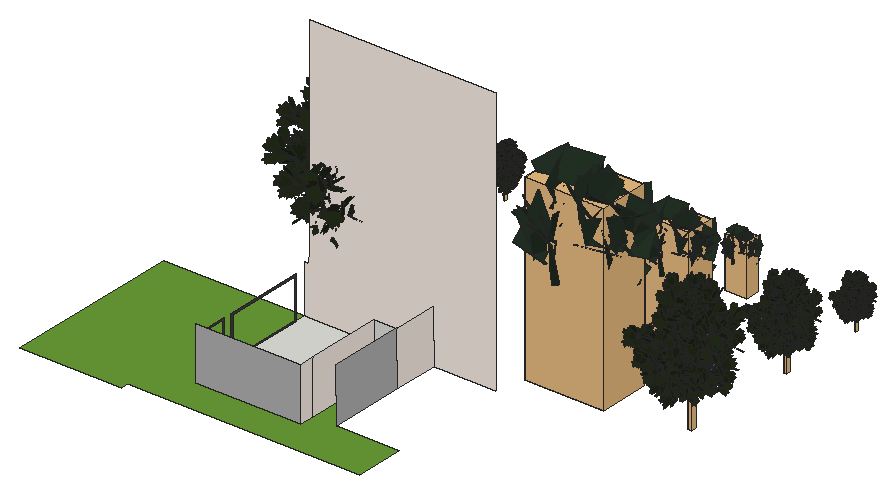
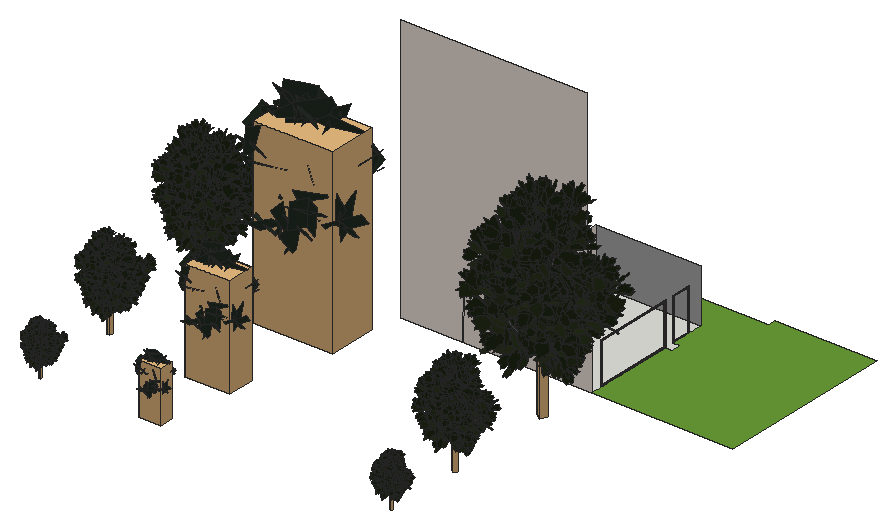
# SketchUp Ruby script. Lengths in inches.
U = 1.inch
M = Sketchup.active_model
def pt(a) = Geom::Point3d.new(a.map { |v| v * U })
def face(e, loops, mat)
  f = e.add_face(loops[0].map { |a| pt(a) })
  loops[1..].each { |l| e.add_face(l.map { |a| pt(a) }).erase! }
  f.material = f.back_material = mat if mat
  f
end
# faces: each face lists its corners as indices into pts; further lists are holes
def faces(e, pts, list, mat = nil) = list.each { |f| face(e, (f[0].is_a?(Array) ? f : [f]).map { |l| l.map { |i| pts[i] } }, mat) }
# xy, xz, yz: faces in a plane at the given z, y or x. An outline is a flat list of corners, or four numbers for a rectangle; further outlines are holes
def ring(l) = l.size == 4 ? [[l[0], l[1]], [l[2], l[1]], [l[2], l[3]], [l[0], l[3]]] : l.each_slice(2).to_a
def flat(e, list, mat, &to3) = list.each { |f| face(e, (f[0].is_a?(Array) ? f : [f]).map { |l| ring(l).map { |u, v| to3.(u, v) } }, mat) }
def xy(e, z, list, mat = nil) = flat(e, list, mat) { |x, y| [x, y, z] }
def xz(e, y, list, mat = nil) = flat(e, list, mat) { |x, z| [x, y, z] }
def yz(e, x, list, mat = nil) = flat(e, list, mat) { |y, z| [x, y, z] }
def lines(e, pts, list) = list.each { |a, b| e.add_line(pt(pts[a]), pt(pts[b])) }
# prism: a flat outline (further loops are holes) pulled along v
def prism(e, loops, v, mat = nil)
  f = face(e, loops, mat); d = Geom::Vector3d.new(v.map { |x| x * U })
  f.pushpull(f.normal.samedirection?(d) ? d.length : -d.length)
end
def box(e, o, s, mat = nil) = prism(e, [[o, [o[0] + s[0], o[1], o[2]], [o[0] + s[0], o[1] + s[1], o[2]], [o[0], o[1] + s[1], o[2]]]], [0, 0, s[2]], mat)
def at(x, y, z, deg = 0) = Geom::Transformation.translation(pt([x, y, z])) * Geom::Transformation.rotation(ORIGIN, Z_AXIS, deg.degrees)
def axes(o, x, y, z) = Geom::Transformation.new([*x, 0, *y, 0, *z, 0, *pt(o).to_a, 1])
def part(name) = M.definitions.add(name)
# library, detail: a bought-in or finely detailed component or shape, given as its bounding box
def library(name, o, s) = part(name).tap { |d| box(d.entities, o, s) }
def detail(e, o, s) = box(e.add_group.entities, o, s)
def put(e, d, t, mat = nil) = e.add_instance(d, t).tap { |i| i.material = mat if mat }
def group(e, t, mat = nil) = e.add_group.tap { |g| g.transformation = t; g.material = mat if mat }.entities
root = M.entities
M.materials.add("Color_D09").color = [86, 59, 49]
M.materials.add("Green ash – green texture").color = [33, 41, 22]
M.materials.add("Niraj_Hair_Gray").color = [178, 178, 178]
M.materials.add("[0009_Linen]").color = [250, 240, 230]
M.materials.add("[Asphalt New]").color = [67, 60, 62]
M.materials.add("[Color_005]1").color = [114, 114, 114]
M.materials.add("[Grass Dark Green]").color = [106, 157, 55]
M.materials.add("euc leaf02").color = [35, 48, 36]
c1 = part("Component\#32")
xz(c1.entities,0,[[2.54,0,9.87,0.64,10.99,2.07,11.4,3.42,15.13,2.28,14.48,4.31,16.14,5.21,16.14,6.08,19.81,7.28,19.6,9.67,17.45,11.49,17.45,12.16,18.82,14.37,17.48,14.37,14.41,13.66,14.41,15.23,12.5625,17.49,9.84,15.21,8.9,13.85,7.74,13.625,7.35,12.68,6.87,13.02,6.35,12.27,5.92,10.47,4.2,7.42,2.84,6.89,0,2.38,0.07,1.59,2.8125,4.94,3.37,3.59,2.54,3.37,2.12,2.22]],"Green ash – green texture")
c2 = part("Component\#31")
xz(c2.entities,0,[[1.1,0,1.61,0,2.73,1.11,4.34,2.72,5.21,6.36,5.85,7.16,6.35,6.9375,6.85,8.05,8.03,8.05,8.625,9.25,10.11,11.7,9.56,13.83,9.56,15.84,7.83,15.84,6.03,14.37,5.31,16.54,4.4375,17.39,1.45,14.31,0,9.15,1.4,5.18,3.01,6.08,1.98,1.39]],"Green ash – green texture")
c3 = part("Component\#30")
put(c3.entities,c1,axes([0,7.77,0],[1,0,0],[0,0.89571,0.44464],[0,-0.44464,0.89571]))
put(c3.entities,c2,axes([2.15,6.37,5.26],[0.57629,-0.80824,0.12095],[0.79263,0.51673,-0.3236],[0.19905,0.28236,0.93843]))
c4 = part("Component\#33")
put(c4.entities,c3,axes([-4.97,-3.22,4.05],[0.69883,-0.69034,0.18725],[0.53248,0.3273,-0.7806],[0.47759,0.64522,0.59632]))
c5 = part("Component\#35")
put(c5.entities,c4,axes([0,5.2,2.2],[1,0,0],[0,0.90259,0.43051],[0,-0.43051,0.90259]))
c6 = part("leaf group 2")
put(c6.entities,c5,axes([-11.99,4.41,-4.35],[2.22014,-0.82385,1.14017],[1.36501,1.77637,-1.37441],[-0.33979,1.75315,1.92841]))
c7 = part("Component\#37")
put(c7.entities,c6,axes([-5.27,11.65,1.68],[-0.48323,0.10636,-0.43072],[-0.11515,-0.64511,-0.03012],[-0.42845,0.05342,0.49388]))
c8 = part("Component\#36")
xz(c8.entities,0,[[0.64,0,0,0.1875,4.21,2.81,8.59,4.11,12.8,4.11,19.57,2.81,12.8,3.73,8.59,3.73,4.21,2.3125]],"Color_D09")
c9 = part("Leaf cluster")
put(c9.entities,c7,axes([23.53,12.57,24.85],[0.06536,-0.90475,-0.42089],[0.61791,-0.2945,0.72901],[-0.78353,-0.30772,0.53981]))
put(c9.entities,c7,axes([22.7,12.25,24.83],[-0.47146,-0.89493,0.11311],[0.80135,-0.48549,-0.35888],[0.36776,-0.0521,0.90651]))
put(c9.entities,c7,axes([24.25,0.65,20.83],[0.8253,-0.50372,0.24924],[0.23848,0.71461,0.65749],[-0.51157,-0.48438,0.71194]))
put(c9.entities,c7,axes([23.54,-2.45,18.63],[0.04689,-0.92492,0.3511],[0.72122,-0.28285,-0.64421],[0.71641,0.2674,0.65188]))
put(c9.entities,c7,axes([22.39,16.15,27.04],[-0.5311,-0.82173,0.2419],[0.41574,0.01583,0.89559],[-0.77461,0.50499,0.40813]))
put(c9.entities,c8,axes([22.76,-5.09,13.48],[0,1.66539,0.44624],[-1.72414,0,0],[0,-0.44624,1.66539]))
c10 = part("Bare twig")
p = [[0,0,0.13],[0.41,0.77,0],[4.07,2.79,10.125],[3.73,2.15,10.23],[7.66,4.77,23.875],[7.4,4.27,23.96],
  [8.6875,5.26,35.99],[8.5,4.91,36.05],[8.32,4.9375,46.95],[8.21,4.74,46.98]]
faces(c10.entities,p,[[0,1,2,3],[3,2,4,5],[4,6,7,5],[6,8,9,7]],"[Color_005]1")
c11 = part("Leafy twig")
put(c11.entities,c10,axes([3.13,0.17,-0.45],[3.38032,6.88592,0.52481],[-5.85488,3.97559,0.303],[0,-1.35912,3.54524]))
put(c11.entities,c7,axes([0.37,31.375,148.94],[0.47772,0.64064,-1.51139],[2.85768,-0.62659,0.20284],[-0.43926,-3.3797,-0.3241]))
c12 = part("Leafy branch")
put(c12.entities,c9,axes([28.11,72.66,46.26],[0.77413,-0.41274,-0.47998],[0.6311,0.56229,0.53435],[0.04934,-0.71657,0.69577]))
put(c12.entities,c9,axes([31.25,3.94,9.17],[0.73236,0.67893,0.05208],[-0.46223,0.55185,-0.69413],[-0.5,0.48428,0.71797]))
put(c12.entities,c9,axes([20.16,84.84,57.95],[0.96628,0.19619,0.16678],[-0.2575,0.73909,0.62245],[-0.00115,-0.6444,0.76469]))
put(c12.entities,c9,axes([30.13,29.18,11.93],[0.86603,0.2796,0.41452],[0,0.82904,-0.55919],[-0.5,0.48428,0.71797]))
put(c12.entities,c9,axes([47.67,28.63,-3.7],[0.1205,-0.71255,0.69119],[0.96646,0.24327,0.08231],[-0.2268,0.65809,0.71797]))
put(c12.entities,c9,axes([48.76,50.64,76.31],[-0.6716,0.46861,-0.57389],[0.01402,0.78248,0.62252],[0.74078,0.41004,-0.53209]))
put(c12.entities,c11,axes([42.34,0,10.34],[0.39368,0,0],[0,0.22544,-0.24092],[0,0.54032,0.50562]))
put(c12.entities,c9,axes([64.51,80.82,101.08],[-0.99604,0.06562,-0.06004],[-0.0106,0.58266,0.81265],[0.08831,0.81006,-0.57966]))
c13 = part("Leafy branch \#2")
put(c13.entities,c9,axes([-3.64,36.17,23.18],[0.95801,0.10249,0.26779],[-0.28581,0.41631,0.86313],[-0.02302,-0.90343,0.42812]))
put(c13.entities,c9,axes([13.16,55.79,39.92],[0.70711,-0.61725,0.34497],[0,0.48786,0.87292],[-0.70711,-0.61725,0.34497]))
put(c13.entities,c11,axes([18.8125,5.17,0.46],[0.25503,0,0],[0,0.20007,-0.0752],[0,0.16866,0.44872]))
put(c13.entities,c9,axes([23.62,-10.17,21.5],[-0.56253,0.81775,0.12181],[0.38738,0.13053,0.91263],[0.73041,0.56057,-0.39021]))
put(c13.entities,c9,axes([45.18,27.18,68.96],[-0.96593,-0.22593,0.12627],[0.12295,0.02876,0.992],[-0.22775,0.97372,0]))
c14 = library("Tree trunk",[-6.35,9.4375,-76.57],[12.56,13.68,315.77])
c15 = part("Leafy branch \#3")
put(c15.entities,c11,axes([21.47,3.93,0.22],[0.25503,0,0],[0,0.21068,-0.03601],[0,0.08077,0.47252]))
put(c15.entities,c9,axes([-4.05,13.6875,55.34],[0.70711,0.70373,-0.069],[0,0.09758,0.99523],[0.70711,-0.70373,0.069]))
put(c15.entities,c9,axes([6.52,33.54,18.07],[0.92587,-0.37604,0.03687],[0,0.09758,0.99523],[-0.37784,-0.92145,0.09035]))
c16 = part("Leafy branch \#1")
put(c16.entities,c9,axes([26.17,74.02,40.56],[0.25882,-0.64004,0.72344],[0,0.74896,0.66262],[-0.96593,-0.1715,0.19384]))
put(c16.entities,c9,axes([6.38,24.03,55.81],[-0.04786,0.8645,-0.50035],[0.15558,0.50126,0.85119],[0.98666,-0.03711,-0.15849]))
put(c16.entities,c11,axes([17.68,0,1.01],[0.32282,0,0],[0,0.21407,-0.16545],[0,0.37107,0.48011]))
put(c16.entities,c9,axes([-9.1875,31.15,28.07],[0.82314,0.37626,-0.42529],[0,0.74896,0.66262],[0.56784,-0.54543,0.61649]))
put(c16.entities,c9,axes([0.54,-12.07,9.94],[0.19622,0.90478,-0.37799],[-0.67396,0.40444,0.61823],[0.71224,0.13344,0.68914]))
put(c16.entities,c9,axes([7.34,9.15,39.57],[0.05153,0.73872,-0.67204],[0.38679,0.60565,0.6954],[0.92072,-0.29578,-0.25452]))
put(c16.entities,c9,axes([36.2,51.23,15.73],[-0.18626,-0.35374,0.91661],[-0.31641,0.90483,0.2849],[-0.93016,-0.23696,-0.28046]))
c17 = part("Tree")
put(c17.entities,c12,axes([209.16,146.26,190.79],[-0.28773,1.46382,-0.87256],[-1.6259,0,0.48096],[0.49836,0.84514,1.51132]))
put(c17.entities,c12,axes([134.38,215.25,141.01],[1.59145,0,0],[0,1.58386,0.23671],[0,-0.32836,1.69393]))
put(c17.entities,c13,axes([178.04,237.71,388.46],[0,-1.63474,0],[1.63474,0,0],[0,0,1.78187]))
put(c17.entities,c12,axes([256.65,171.18,211.31],[-1.36815,1.04036,0],[-1.04036,-1.36815,0],[0,0,1.87346]))
put(c17.entities,c12,axes([167.11,160.33,284.63],[0.63716,1.20925,-0.47341],[-1.25908,0.71729,0.13762],[0.43501,0.34501,1.46674]))
put(c17.entities,c14,axes([199.97,188.06,127.43],[1.59145,0,0],[0,1.59145,0],[0,0,1.66425]))
put(c17.entities,c12,axes([275.77,218.4,281.93],[-1.57517,-0.28132,-0.44593],[0.06295,-1.50318,0.62621],[-0.42383,0.67416,1.53786]))
put(c17.entities,c12,axes([190.14,288,146.64],[0.35111,-1.78964,0],[1.72866,0.33915,0.47202],[-0.50488,-0.09905,1.92016]))
put(c17.entities,c12,axes([257.54,236.65,165.53],[-1.29152,-0.54158,0],[0.54158,-1.29152,0],[0,0,1.52652]))
put(c17.entities,c12,axes([175.36,274.13,265.04],[0.47642,-1.31213,-0.12271],[1.30597,0.45529,0.24003],[-0.16973,-0.17989,1.50253]))
put(c17.entities,c13,axes([228.65,212.14,385.35],[-1.53723,0.39369,-0.12111],[-0.39786,-1.55122,0.00748],[-0.10661,0.11241,1.71849]))
put(c17.entities,c15,axes([179.375,247.82,455.73],[0.79573,-1.37824,0],[1.37824,0.79573,0],[0,0,1.73468]))
put(c17.entities,c15,axes([220.2,190.4,436.52],[-0.90108,1.29724,0.19482],[-1.26794,-0.9219,0.27414],[0.36658,0,1.69551]))
put(c17.entities,c16,axes([195.4,185.625,330.61],[0,1.80471,0],[-1.731,0,0.5105],[0.55644,0,1.88679]))
put(c17.entities,c16,axes([180.07,237.23,322.66],[1.03006,-1.73903,-0.39964],[1.71651,0.8636,0.79163],[-0.4607,-0.67055,2.05597]))
put(c17.entities,c12,axes([252.86,167.09,121.2],[-1.29065,1.04142,0.30989],[-1.03312,-1.28343,0.15838],[0.47872,-0.11505,1.68865]))
put(c17.entities,c12,axes([145.45,238.15,252.03],[1.32497,-0.45364,0],[0.45364,1.32497,0],[0,0,1.52652]))
put(c17.entities,c16,axes([222.54,228.83,294],[-1.20488,-1.04179,0.83261],[1.23186,-1.24114,0.27288],[0.38905,0.70343,1.7146]))
put(c17.entities,c16,axes([223.77,224.36,314.875],[-1.40575,-0.68986,-0.30962],[0.56266,-1.37824,0.6133],[-0.4899,0.39658,1.59284]))
put(c17.entities,c16,axes([166.75,216.1,346.53],[1.65511,0,0],[0,1.6365,0.2475],[0,-0.26977,1.78379]))
put(c17.entities,c13,axes([162.33,209.39,372.71],[1.56679,-0.27909,0],[0.27909,1.56679,0],[0,0,1.73468]))
put(c17.entities,c13,axes([203.35,171.86,386.35],[0.15996,1.63137,0],[-1.63137,0.15996,0],[0,0,1.78672]))
c18 = part("Green Ash")
put(c18.entities,c14,axes([99.99,94.03,63.71],[0.79573,0,0],[0,0.79573,0],[0,0,0.83213]))
put(c18.entities,c13,axes([101.67,85.93,193.17],[0.07998,0.81569,0],[-0.81569,0.07998,0],[0,0,0.89336]))
put(c18.entities,c13,axes([89.02,118.86,194.23],[0,-0.81737,0],[0.81737,0,0],[0,0,0.89093]))
put(c18.entities,c12,axes([137.88,109.2,140.96],[-0.78759,-0.14066,-0.22296],[0.03147,-0.75159,0.31311],[-0.21191,0.33708,0.76893]))
put(c18.entities,c12,axes([67.1875,107.625,70.5],[0.79573,0,0],[0,0.79193,0.11835],[0,-0.16418,0.84696]))
put(c18.entities,c12,axes([104.58,73.13,95.39],[-0.14386,0.73191,-0.43628],[-0.81295,0,0.24048],[0.24918,0.42257,0.75566]))
put(c18.entities,c12,axes([128.33,85.59,105.66],[-0.68407,0.52018,0],[-0.52018,-0.68407,0],[0,0,0.93673]))
put(c18.entities,c12,axes([128.77,118.32,82.77],[-0.64576,-0.27079,0],[0.27079,-0.64576,0],[0,0,0.76326]))
put(c18.entities,c13,axes([114.32,106.07,192.67],[-0.76861,0.19684,-0.06056],[-0.19893,-0.77561,0.00374],[-0.0533,0.05621,0.85925]))
put(c18.entities,c12,axes([83.56,80.16,142.32],[0.31858,0.60462,-0.23671],[-0.62954,0.35865,0.06881],[0.21751,0.1725,0.73337]))
put(c18.entities,c13,axes([81.16,104.7,186.36],[0.7834,-0.13954,0],[0.13954,0.7834,0],[0,0,0.86734]))
put(c18.entities,c16,axes([97.7,92.8125,165.31],[0,0.90235,0],[-0.8655,0,0.25525],[0.27822,0,0.94339]))
put(c18.entities,c12,axes([87.68,137.07,132.52],[0.23821,-0.65607,-0.06135],[0.65299,0.22764,0.12002],[-0.08486,-0.08995,0.75126]))
put(c18.entities,c15,axes([89.6875,123.91,227.86],[0.39786,-0.68912,0],[0.68912,0.39786,0],[0,0,0.86734]))
put(c18.entities,c12,axes([95.07,144,73.32],[0.17556,-0.89482,0],[0.86433,0.16957,0.23601],[-0.25244,-0.04953,0.96008]))
put(c18.entities,c15,axes([110.1,95.2,218.26],[-0.45054,0.64862,0.09741],[-0.63397,-0.46095,0.13707],[0.18329,0,0.84775]))
put(c18.entities,c16,axes([90.03,118.62,161.33],[0.51503,-0.86951,-0.19982],[0.85825,0.4318,0.39581],[-0.23035,-0.33528,1.02798]))
put(c18.entities,c16,axes([83.38,108.05,173.27],[0.82756,0,0],[0,0.81825,0.12375],[0,-0.13489,0.89189]))
put(c18.entities,c16,axes([111.27,114.42,147],[-0.60244,-0.5209,0.41631],[0.61593,-0.62057,0.13644],[0.19452,0.35171,0.8573]))
put(c18.entities,c12,axes([126.43,83.55,60.6],[-0.64533,0.52071,0.15494],[-0.51656,-0.64172,0.07919],[0.23936,-0.05752,0.84432]))
put(c18.entities,c16,axes([111.89,112.18,157.4375],[-0.70287,-0.34493,-0.15481],[0.28133,-0.68912,0.30665],[-0.24495,0.19829,0.79642]))
put(c18.entities,c12,axes([72.73,119.08,126.01],[0.66249,-0.22682,0],[0.22682,0.66249,0],[0,0,0.76326]))
c19 = library("Group\#99",[0,0,0],[259.75,161.77,589.29])
c20 = part("Blue Gum")
p = [[271.53,158.18,378.25],[270.5625,158.71,380.69],[270.37,158.83,381.17],[272.73,162.06,384.51],[213.85,150.08,152.75],[212.24,149.06,149.65],
  [150.49,110.24,344.32],[151.97,108.18,342.21],[217.47,152.58,206.91],[209.32,150.04,213.6],[153.27,112.37,338.72],[213.34,156.04,223.13],
  [212.17,155.27,219.89],[213.66,148.52,337.14],[212.6875,151.94,345.88],[201.33,160.36,0],[198.82,151.26,0.01],[228.58,150.59,468.55],
  [228.91,150.53,474.28],[226.95,148.99,472.86]]
faces(c20.entities,p,[[0,1,2],[1,0,3],[3,2,1]])
lines(c20.entities,p,[[4,5],[6,7],[8,9],[10,6],[7,10],[11,12],[13,14],[15,16],[17,18],[19,17],[18,19]])
put(c20.entities,c19,axes([324.42,234.92,0.08],[-1,0,-0.00067],[0,-1,0.00003],[-0.00067,0.00003,1]))
g1 = group(c20.entities,at(392.72,299.04,214.24))
p = [[-190.24,-45.24,49.75],[-155.8,-83.51,-0.1],[-171.1,-117.4,15.86],[-186.4,-151.3,31.82],[-220.85,-113.03,81.67],[-197.84,-62.08,57.68],
  [-156.97,-85.38,90],[-134.58,-101.98,23.98],[-207.62,-132.83,7.74],[-230.01,-116.24,73.77],[-175.11,-93.05,85.97],[-155.875,-47.35,89.82],
  [-171.875,-81.0625,28.63],[-175.09,-115.85,49.06],[-178.3125,-150.63,69.48],[-162.3125,-116.92,130.67],[-157.47,-64.63,99.96],[-108.86,-93.44,91.87],
  [-142.19,-103.1875,29.18],[-207.99,-128.51,68.93],[-174.66,-118.76,131.62],[-125.2,-99.73,101.74],[-105.25,-143.93,101.02],[-118.65,-122.91,33.83],
  [-139.46,-91.34,48.24],[-160.28,-59.76,62.65],[-146.87,-80.78,129.84],[-115.59,-128.24,108.18],[-69.65,-64.39,98.91],[-102.98,-74.13,36.22],
  [-135.88,-86.79,56.09],[-168.78,-99.45,75.97],[-135.45,-89.7,138.66],[-85.99,-70.68,108.78],[-206,0,112.1],[-205.51,-55.1,41.09],
  [-219.69,-93.37,71.26],[-233.87,-131.63,101.43],[-234.36,-76.53,172.4375],[-220.18,-38.26,142.27],[-213.05,-19.01,127.09],[-58.99,-92.56,99.73],
  [-109.77,-114.37,54.1],[-132.54,-82.69,64.86],[-155.3,-51.01,75.61],[-104.53,-29.2,121.24],[-70.31,-76.82,105.07],[-84.85,-14.67,104.44],
  [-93.72,-70.0625,59.84],[-130.5,-76.32,75.5],[-167.29,-82.57,91.16],[-158.42,-27.18,135.76],[-103.12,-17.78,112.22],[-170.99,-48.24,149.78],
  [-170.5,-103.34,78.77],[-268.88,-83.39,63.75],[-269.37,-28.29,134.76],[-195.43,-43.28,146.05],[-119.44,-162.62,158.17],[-165.08,-157.98,109.24],
  [-139.69,-139.86,87.75],[-114.31,-121.74,66.26],[-68.68,-126.38,115.19],[-94.0625,-144.5,136.68],[-106.83,-153.62,147.5],[-83.43,-178.22,123.11],
  [-129.0625,-173.58,74.18],[-150.32,-106.13,101.32],[-104.69,-110.78,150.25],[-88.71,-161.47,129.85],[-153.18,-33.52,154.23],[-187.55,-61.6,76.08],
  [-205.14,-103.18,99.27],[-222.72,-144.75,122.47],[-188.35,-116.67,200.62],[-170.77,-75.09,177.42],[-161.92,-54.17,165.75],[-126.95,-97.9375,165.85],
  [-161.32,-126.02,87.7],[-248.95,-80.33,110.85],[-214.58,-52.25,189],[-148.72,-86.59,171.6],[-365.27,-93.53,149.96],[-339.43,-156.16,87.91],
  [-290.4375,-139.67,92.34],[-241.45,-123.17,96.77],[-267.29,-60.54,158.83],[-340.93,-85.33,152.16],[-220,-209.94,88.83],[-192.18,-284.625,134.55],
  [-202.3,-275.33,156.35],[-232.93,-247.2,222.33],[-260.75,-172.52,176.61],[-240.375,-191.23,132.72],[-392.72,-100.24,198.19],[-366.88,-162.88,136.14],
  [-328.26,-131.57,121.3],[-289.64,-100.27,106.47],[-315.48,-37.63,168.52],[-373.54,-84.69,190.82],[-327.95,-161.62,221.67],[-317.1,-180.89,132.49],
  [-328.31,-131.57,120.9375],[-339.53,-82.25,109.39],[-350.38,-62.97,198.5625],[-333.52,-137.11,215.93],[-255.83,-236.76,152.47],[-329.61,-198.39,191.52],
  [-323.5,-175.58,181.2],[-305,-106.55,149.96],[-231.21,-144.93,110.9],[-243.52,-190.85,131.6875],[-205.5,-81.8,220.89],[-197.86,-85.86,131.43],
  [-243.5,-64.11,127],[-289.13,-42.35,122.57],[-296.77,-38.29,212.03],[-251.13,-60.04,216.46],[-228.17,-70.99,218.6875],[-234.33,-241.65,142.48],
  [-225.25,-222.09,231.79],[-228.94,-197.05,226.92],[-240.1,-121.29,212.17],[-249.18,-140.85,122.86],[-241.75,-191.25,132.67],[-227.68,-15.04,215.96],
  [-220.04,-19.1,126.5],[-266.95,-109.11,127.5],[-274.59,-105.04,216.95],[-239.33,-37.4,216.21],[-312.18,-35.14,201.88],[-307.82,-106.7,144.42],
  [-256.66,-99.36,139.9],[-205.5,-92.02,135.375],[-209.86,-20.46,192.83],[-286.77,-31.49,199.63],[-224.25,-107.3,143.78],[-158.47,-57.42,184.1],
  [-153.89,-76.52,200.79],[-140.05,-134.32,251.29],[-205.83,-184.2,210.96],[-215.04,-145.75,177.37],[-371.18,-63.42,218.95],[-318.87,-74.08,144.18],
  [-278.67,-86.3125,174.61],[-238.47,-98.55,205.04],[-290.78,-87.88,279.82],[-351.21,-69.49,234.07],[-314.82,-59.28,247.3],[-323.0625,-96.32,163.62],
  [-272.16,-89.61,156.15],[-221.26,-82.9,148.67],[-213.02,-45.87,232.35],[-289.54,-55.95,243.59],[-269.6,-260.65,169.64],[-261.02,-289.45,256.47],
  [-255.15,-265.53,264.0625],[-237.36,-193.15,287.04],[-245.94,-164.36,200.22],[-257.77,-212.5,184.93],[-219.98,-94.58,184.38],[-135.38,-92.14,220.14],
  [-132.93,-117.5625,216.66],[-125.5,-194.48,206.12],[-210.1,-196.92,170.36],[-242.72,-259.5,171.19],[-311.27,-292.91,222.44],[-317.8125,-269.04,229.65],
  [-337.62,-196.84,251.48],[-269.07,-163.43,200.23],[-255.89,-211.46,185.71],[-204.01,-188.2,177.79],[-188.33,-208.64,265.98],[-194.51,-184.59,272.89],
  [-213.23,-111.83,293.8125],[-228.92,-91.39,205.62],[-216.46,-139.79,191.7],[-111.12,-172.19,178.4],[-144.16,-223.61,247],[-146.96,-202.62,261.69],
  [-155.45,-139.1,306.14],[-122.41,-87.68,237.53],[-116.76,-129.9375,207.97],[-92.3,-219.25,321.53],[-140.07,-175.86,256.125],[-105.48,-191.84,220.91],
  [-70.89,-207.83,185.69],[-23.13,-251.22,251.1],[-75.12,-227.1875,304.03],[-95.32,-86.56,260.02],[-28.15,-67.53,258.27],[-24.95,-79.6,243.18],
  [-15.25,-116.11,197.51],[-82.42,-135.13,199.26],[-88.87,-110.84,229.64],[-230.35,-182.42,199.75],[-240.26,-200.67,289.25],[-235.09,-176.09,295.07],
  [-219.44,-101.74,312.67],[-209.53,-83.5,223.17],[-219.9375,-132.96,211.46],[-140.68,-151.65,266.01],[-78.24,-142.94,332.84],[-63.08,-129.17,317.2],
  [-17.2,-87.5,269.85],[-79.64,-96.22,203.02],[-110.16,-123.93,234.52],[-181.78,-155.46,254.29],[-197.87,-106.1875,330.15],[-215.8125,-92.48,317.72],
  [-270.1,-51.01,280.11],[-254.02,-100.28,204.25],[-217.9,-127.875,229.27],[-219.05,-237.83,228.68],[-246.19,-265.11,312.11],[-270.4375,-258.25,306.72],
  [-343.82,-237.49,290.4],[-316.68,-210.21,206.96],[-267.86,-224.02,217.82],[-221.64,-245.99,220.16],[-255.74,-296.14,289.1875],[-278.74,-284.87,286.3125],
  [-348.35,-250.78,277.61],[-314.25,-200.64,208.59],[-267.95,-223.32,214.37],[-214.08,-176.63,246.6],[-287.9,-162.75,299.5],[-289.8,-138.53,290.89],
  [-295.55,-65.24,264.85],[-221.72,-79.12,211.94],[-273.56,-277.41,225.52],[-332.72,-264.05,294.53],[-330.67,-238.52,291.65],[-324.47,-161.27,282.95],
  [-265.3,-174.62,213.93],[-269.43,-226.01,219.72],[-125.42,-280.5,273.74],[-154.49,-208.42,224.74],[-56.47,-175.26,217.08],[-27.39,-247.34,266.08],
  [-101.07,-272.26,271.84],[-137.08,-126.63,220.68],[-181.31,-63.4,270.55],[-159.07,-51.25,275.29],[-91.8,-14.51,289.63],[-47.57,-77.74,239.76],
  [-92.33,-102.1875,230.22],[-238.16,-243.49,222.62],[-218.34,-248.07,312.22],[-217.08,-222.36,313.49],[-213.28,-144.56,317.34],[-233.09,-139.97,227.74],
  [-235.625,-191.73,225.18],[-96.8,-128.7,236.99],[-25.62,-162.74,224.18],[-29.7,-177.8,240.28],[-42.05,-223.37,289.02],[-113.23,-189.33,301.82],
  [-105.01,-159.01,269.41],[-190.11,-164.1875,296.41],[-166.86,-101.93,340.84],[-154.3,-94.29,323.91],[-116.3,-71.16,272.67],[-139.55,-133.41,228.25],
  [-164.83,-148.8,262.33],[-190.89,-165.45,228.74],[-213.01,-227.55,273.96],[-199.51,-220.6,290.46],[-158.68,-199.56,340.39],[-136.56,-137.46,295.18],
  [-163.73,-151.45,261.96],[-108.84,-65.86,242.35],[-143.91,-74.96,326.78],[-145.22,-100.52,323.73],[-149.17,-177.86,314.51],[-114.09,-168.76,230.08],
  [-111.47,-117.3125,236.21],[-131.79,-76.12,256.875],[-89.01,-36.19,327.71],[-66.95,-47.86,321.26],[-0.2,-83.16,301.74],[-42.99,-123.09,230.91],
  [-87.39,-99.61,243.89],[-191.96,-179.86,282.46],[-135.02,-196.07,336.18],[-121.21,-181.46,326.24],[-79.42,-137.25,296.18],[-136.36,-121.05,242.47],
  [-164.16,-150.45,262.47],[-230.13,-253.21,246.97],[-260.13,-299.04,320.74],[-267.04,-276.89,331.97],[-287.96,-209.88,365.95],[-257.97,-164.06,292.17],
  [-244.05,-208.64,269.57],[-280.97,-237.22,246.96],[-334.39,-225.07,320.72],[-316.05,-210.87,331.95],[-260.54,-167.9,365.9375],[-207.12,-180.05,292.18],
  [-123.3,-254.01,336.04],[-125.12,-228.29,247.85],[-81.63,-201.01,255.39],[-38.14,-173.74,262.92],[-36.32,-199.46,351.11],[-101.69,-240.46,339.78],
  [-68.26,-134.5,260.14],[-26.24,-201.97,251.74],[-44.5,-214.15,256.34],[-99.74,-251,270.27],[-141.76,-183.53,278.67],[-121.3,-170.4,347.79],
  [-129.86,-181.96,257.04],[-33.4,-220.07,253.73],[-24.85,-208.51,344.48],[-97.34,-179.87,346.97],[-78.09,-121.04,341.08],[-129.1,-143.71,268.11],
  [-128.64,-193.18,283.74],[-128.18,-242.65,299.36],[-77.17,-219.98,372.34],[-77.86,-145.61,348.85],[-177.42,-71.46,329.51],[-152.53,-122.65,273.39],
  [-155.7,-156.33,303.27],[-158.88,-190.01,333.16],[-183.78,-138.82,389.27],[-179,-88.19,344.35],[-150.51,-90.39,274.04],[-160.0625,-83.41,365.16],
  [-137.04,-94.48,368.65],[-67.4,-127.95,379.21],[-57.85,-134.93,288.09],[-104.18,-112.66,281.07],[-94.02,-187.3,327.96],[-81.13,-138.55,389.98],
  [-69.09,-124.83,376.95],[-32.66,-83.33,337.53],[-45.54,-132.09,275.51],[-69.78,-159.69,301.74],[-118.35,-128.14,277.49],[-134.07,-116.2,367.22],
  [-118.18,-95.9,367.54],[-70.12,-34.49,368.49],[-54.4,-46.4375,278.76],[-86.375,-87.29,278.12],[-130.67,-185.64,278.8125],[-99.69,-223.89,341.79],
  [-81.85,-210.3,341.52],[-27.87,-169.2,340.6875],[-58.85,-130.95,277.71],[-94.76,-158.29,278.26],[-124.09,-168.51,302.87],[-98.25,-187.53,376.08],
  [-77.34,-181.72,370.43],[-14.08,-164.14,353.32],[-39.93,-145.12,280.11],[-82.01,-156.82,291.49],[-222.9,-199.13,376.1],[-220.07,-149.45,341.44],
  [-227.34,-168.57,313.98],[-234.62,-187.6875,286.52],[-237.45,-237.37,321.18],[-230.17,-218.25,348.64],[-226.51,-208.63,362.46],[-66.91,-203,314.13],
  [-2.98,-185.26,358.72],[-4.41,-163.74,352.56],[-8.73,-98.64,333.94],[-72.66,-116.39,289.35],[-169.41,-164.76,388.4],[-177.97,-176.3125,297.65],
  [-129.74,-195.37,296],[-81.52,-214.43,294.34],[-72.96,-202.87,385.09],[-145.46,-174.22,387.58],[-154.72,-129.21,384.88],[-129.15,-146.67,298.38],
  [-129.71,-197.46,308.96],[-130.27,-248.25,319.53],[-155.84,-230.78,406.04],[-155,-154.4375,390.14],[-202.43,-168.15,321.54],[-179.78,-204.63,388.96],
  [-158.3,-199.98,384.5],[-93.32,-185.9,371.01],[-115.96,-149.42,303.58],[-159.19,-158.79,312.5625],[-197.46,-225.01,341.1],[-194.63,-175.33,306.4375],
  [-260.05,-161.8125,321.53],[-262.88,-211.49,356.1875],[-213.71,-221.65,344.85],[-157.48,-194.21,341.46],[-113.86,-228.8,398.82],[-95.37,-218.73,391.1],
  [-39.42,-188.27,367.76],[-83.04,-153.67,310.41],[-120.26,-173.9375,325.9375],[-193.32,-187.43,311.78],[-211.98,-162.83,385.51],[-194.23,-149.13,385.64],
  [-140.53,-107.67,386.06],[-121.86,-132.27,312.33],[-157.59,-159.85,312.05],[-258.44,-158.87,437.95],[-244.84,-121.05,355.33],[-234.18,-168.04,336.09],
  [-223.52,-215.03,316.85],[-237.12,-252.84,399.47],[-253.15,-182.21,428.39],[-193.45,-225.28,404.25],[-172.56,-175.18,330.125],[-129.23,-203.0625,324.0625],
  [-85.9,-230.95,318],[-106.8,-281.05,392.12],[-171.93,-239.14,401.24],[-189.32,-183.99,368.07],[-165.25,-149.36,435.97],[-148.5625,-139.1,425.06],
  [-98.07,-108.05,392.03],[-122.15,-142.68,324.13],[-155.73,-163.33,346.1],[-155.65,-206.76,334.06],[-167.83,-218.04,412.25],[-167.96,-195.875,415.63],
  [-168.38,-128.8,425.86],[-156.21,-117.52,347.67],[-155.93,-162.14,340.86],[-145.4375,-206.81,336.52],[-133.41,-216.07,415],[-138.07,-194.41,418.47],
  [-152.15,-128.87,428.97],[-164.18,-119.61,350.49],[-154.81,-163.21,343.5],[-277.65,-112.64,443.48],[-209.06,-142.23,389.99],[-242.625,-172.43,364.44],
  [-276.2,-202.63,338.89],[-344.79,-173.04,392.38],[-294.33,-127.64,430.79],[-116.84,-180.91,416.6],[-166.69,-214.06,346.91],[-201.41,-176.24,354.36],
  [-236.13,-138.41,361.82],[-186.28,-105.26,431.51],[-134.09,-162.12,420.31],[-150.67,-209.23,358.7],[-156.56,-222.56,437.29],[-138.24,-210.16,440.97],
  [-82.8125,-172.64,452.1],[-76.93,-159.31,373.5],[-113.8,-184.27,366.1],[-154.14,-165.42,373.5],[-127.09,-136.44,442.91],[-107.04,-145.81,439.23],
  [-46.4,-174.14,428.11],[-73.46,-203.11,358.7],[-161.71,-108.91,440.68],[-158.5,-155.86,361.76],[-202.41,-180.14,374.96],[-246.32,-204.43,388.15],
  [-249.52,-157.48,467.07],[-183.52,-120.98,447.23]]
faces(g1,p,[[0,1,2,3,4,5],[6,7,2,8,9,10],[11,12,13,14,15,16],[17,18,13,19,20,21],[22,23,24,25,26,27],[28,29,30,31,32,33],[34,35,36,37,38,39,40],[41,42,43,44,45,46],
  [47,48,49,50,51,52],[53,54,36,55,56,39,57],[58,59,60,61,62,63,64],[65,66,60,67,68,63,69],[70,71,72,73,74,75,76],[77,78,72,79,80,75,81],[82,83,84,85,86,87],[88,89,90,91,92,93],
  [94,95,96,97,98,99],[100,101,102,103,104,105],[106,107,108,109,110,111],[112,113,114,115,116,117,118],[119,120,121,122,123,124],[125,126,114,127,128,117,129],[130,131,132,133,134,135],[136,137,138,139,140,141],
  [142,143,144,145,146,147],[148,149,150,151,152,153],[154,155,156,157,158,159],[160,161,162,163,164,141],[165,166,167,168,169,170],[171,172,173,174,175,176],[177,178,179,180,181,182],[183,184,185,186,187,188],
  [189,190,191,192,193,194],[195,196,197,198,199,200],[201,202,203,204,205,206],[207,208,209,210,211,212],[213,214,215,216,217,218],[219,220,221,222,223,224],[225,226,227,228,229,212],[230,231,232,233,234,235],
  [236,237,185,238,239,240],[241,242,243,244,245,246],[247,248,249,250,251,252],[253,254,255,256,257,258],[259,260,261,262,263,264],[265,266,267,268,269,270],[271,272,273,274,275,276],[277,278,279,280,281,282],
  [283,284,285,286,287,288],[289,290,291,292,293,294],[295,296,297,298,299,294],[300,301,302,303,304,305],[306,307,308,309,310,258],[311,312,302,313,314,315],[316,317,318,319,320,321],[322,323,324,325,326,327],
  [328,329,330,331,332,333],[334,335,336,337,338,339],[340,341,342,343,344,345],[346,347,348,349,350,351],[352,353,354,355,356,357],[358,359,360,361,362,363,364],[365,366,367,368,369,339],[370,371,372,373,374,375],
  [376,377,378,379,380,381],[382,383,384,385,386,387],[388,389,360,390,391,363,392],[393,394,395,396,397,398],[399,400,401,402,403,404],[405,406,407,408,409,410],[411,412,413,414,415,416],[417,418,419,420,421,422],
  [423,424,425,426,427,428],[429,430,431,432,433,434],[435,436,437,438,439,440],[441,442,443,444,445,446],[447,448,449,450,451,452],[453,454,455,456,457,452],[458,459,460,461,462,463]],"euc leaf02")
xy(root,0,[[597.61,153,836.65,153,836.65,360.375,882.97,360.375,882.97,464.11,597.61,464.11,597.61,254.44,582.23,254.44,582.23,233.07,597.61,233.07],[882.97,360.375,890.84,464.11]])
xy(root,0,[[275.09,57.05,506.24,57.05,506.24,75.24,1032.97,75.24,1032.97,187.625,890.84,187.625,890.84,360.375,836.65,360.375,836.65,153,597.61,153,597.61,233.07,582.23,233.07,582.23,254.44,597.61,254.44,597.61,464.11,275.09,464.11]],"[Grass Dark Green]")
xz(root,153,[[597.61,0,836.65,121.74]],"Niraj_Hair_Gray")
xz(root,360.375,[[836.65,0,890.84,0,888.76,121.74,836.65,121.74]])
xz(root,464.11,[[597.61,0,597.61,109.91,607.36,109.91,607.36,121.74,608.47,121.74,608.47,607.875,1032.97,607.875,1032.97,0]],"[0009_Linen]")
yz(root,597.61,[[[186.88,0,233.07,97.1875],[189.81,2.93,230.14,94.26]],[[254.44,0,437.85,97.125],[258.06,3.62,434.24,93.51]]],"[Asphalt New]")
yz(root,836.65,[[153,0,187.625,121.74],[187.625,0,360.375,121.74]],"[0009_Linen]")
p = [[888.71,187.625,124.25],[888.71,360.375,124.25],[888.76,360.375,121.74],[890.84,360.375,0],[890.84,187.625,0],[890.84,464.11,0],
  [888.76,464.11,121.74]]
faces(root,p,[[0,1,2,3,4]],"Niraj_Hair_Gray")
faces(root,p,[[2,3,5,6]],"[0009_Linen]")
put(root,c17,axes([663.6,366.75,0],[0.42475,0.62972,0],[-0.62972,0.42475,0],[0,0,0.75958]))
put(root,c18,at(1290.13,468.08,0))
put(root,c17,axes([635.95,728.99,0],[0.21238,0.31486,0],[-0.31486,0.21238,0],[0,0,0.37979]))
put(root,c18,axes([1331.18,765.7,2.93],[0.66,0,0],[0,0.66,0],[0,0,0.66]))
put(root,c18,axes([1358.14,993.15,-0.07],[0.3828,0,0],[0,0.3828,0],[0,0,0.3828]))
put(root,c17,axes([624.5,961.79,0],[0.10619,0.15743,0],[-0.15743,0.10619,0],[0,0,0.1899]))
put(root,c20,axes([1000.61,477.37,-0.03],[0.7,0,0],[0,0.7,0],[0,0,0.7]))
put(root,c20,axes([1071.78,777.6,-0.06],[0.392,0,0],[0,0.392,0],[0,0,0.392]))
put(root,c20,axes([1108.63,989.52,-0.08],[0.196,0,0],[0,0.196,0],[0,0,0.196]))
